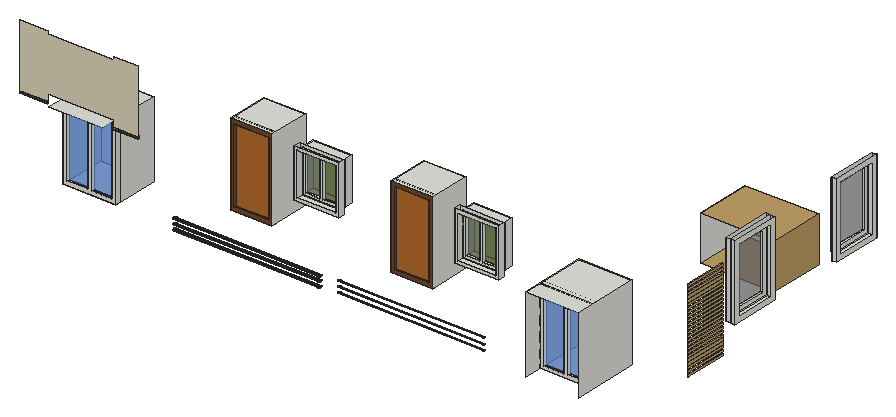
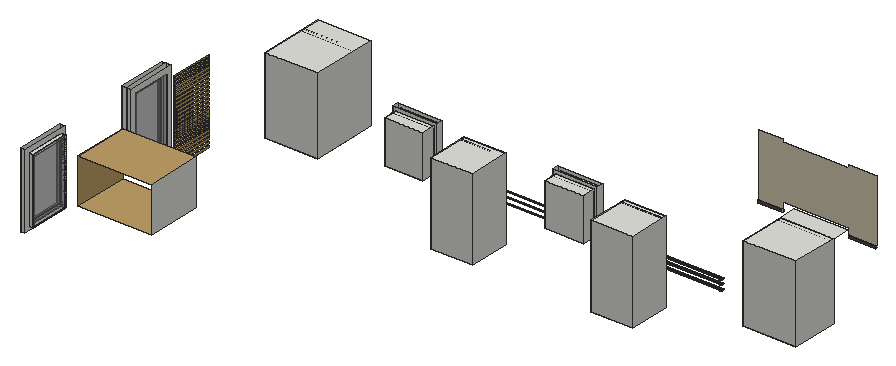
# SketchUp Ruby script. Lengths in inches.
U = 1.inch
M = Sketchup.active_model
def pt(a) = Geom::Point3d.new(a.map { |v| v * U })
def face(e, loops, mat)
  f = e.add_face(loops[0].map { |a| pt(a) })
  loops[1..].each { |l| e.add_face(l.map { |a| pt(a) }).erase! }
  f.material = f.back_material = mat if mat
  f
end
# faces: each face lists its corners as indices into pts; further lists are holes
def faces(e, pts, list, mat = nil) = list.each { |f| face(e, (f[0].is_a?(Array) ? f : [f]).map { |l| l.map { |i| pts[i] } }, mat) }
# xy, xz, yz: faces in a plane at the given z, y or x. An outline is a flat list of corners, or four numbers for a rectangle; further outlines are holes
def ring(l) = l.size == 4 ? [[l[0], l[1]], [l[2], l[1]], [l[2], l[3]], [l[0], l[3]]] : l.each_slice(2).to_a
def flat(e, list, mat, &to3) = list.each { |f| face(e, (f[0].is_a?(Array) ? f : [f]).map { |l| ring(l).map { |u, v| to3.(u, v) } }, mat) }
def xy(e, z, list, mat = nil) = flat(e, list, mat) { |x, y| [x, y, z] }
def xz(e, y, list, mat = nil) = flat(e, list, mat) { |x, z| [x, y, z] }
def yz(e, x, list, mat = nil) = flat(e, list, mat) { |y, z| [x, y, z] }
def lines(e, pts, list) = list.each { |a, b| e.add_line(pt(pts[a]), pt(pts[b])) }
# prism: a flat outline (further loops are holes) pulled along v
def prism(e, loops, v, mat = nil)
  f = face(e, loops, mat); d = Geom::Vector3d.new(v.map { |x| x * U })
  f.pushpull(f.normal.samedirection?(d) ? d.length : -d.length)
end
def box(e, o, s, mat = nil) = prism(e, [[o, [o[0] + s[0], o[1], o[2]], [o[0] + s[0], o[1] + s[1], o[2]], [o[0], o[1] + s[1], o[2]]]], [0, 0, s[2]], mat)
def at(x, y, z, deg = 0) = Geom::Transformation.translation(pt([x, y, z])) * Geom::Transformation.rotation(ORIGIN, Z_AXIS, deg.degrees)
def axes(o, x, y, z) = Geom::Transformation.new([*x, 0, *y, 0, *z, 0, *pt(o).to_a, 1])
def part(name) = M.definitions.add(name)
# library, detail: a bought-in or finely detailed component or shape, given as its bounding box
def library(name, o, s) = part(name).tap { |d| box(d.entities, o, s) }
def detail(e, o, s) = box(e.add_group.entities, o, s)
def put(e, d, t, mat = nil) = e.add_instance(d, t).tap { |i| i.material = mat if mat }
def group(e, t, mat = nil) = e.add_group.tap { |g| g.transformation = t; g.material = mat if mat }.entities
root = M.entities
M.materials.add("Generic").color = [191, 159, 103]
M.materials.add("Generic\#3").color = [218, 209, 183]
M.materials.add("[Color M06]").color = [86, 86, 86]
M.materials.add("[Translucent Glass Blue]").color = [100, 149, 237]
M.materials["[Translucent Glass Blue]"].alpha = 0.5
M.materials.add("[Translucent Glass Dark Green]").color = [62, 91, 5]
M.materials["[Translucent Glass Dark Green]"].alpha = 0.5
M.materials.add("[Translucent Glass Gray]").color = [128, 128, 128]
M.materials["[Translucent Glass Gray]"].alpha = 0.5
M.materials.add("[Wood Bamboo]").color = [177, 105, 43]
M.materials.add("[Wood Veneer 01]").color = [120, 70, 37]
c1 = part("Group\#5")
xy(c1.entities,0,[[0,0,1,57.75]])
xy(c1.entities,2.57,[[0,0,1,57.75]])
xz(c1.entities,0,[[0,0,1,2.57]])
xz(c1.entities,57.75,[[0,0,1,2.57]])
yz(c1.entities,1,[[0,0,57.75,2.57]])
c2 = part("Group\#4")
xy(c2.entities,0,[[0,0,55.6875,6]],"[Wood Veneer 01]")
xy(c2.entities,4.75,[[4.75,0,50.9375,3]],"[Wood Veneer 01]")
xy(c2.entities,105.5,[[4.75,0,50.9375,3]],"[Wood Veneer 01]")
xy(c2.entities,110.25,[[0,0,55.6875,6]],"[Wood Veneer 01]")
xz(c2.entities,0,[[[0,0,55.6875,110.25],[4.75,4.75,50.9375,105.5]]],"[Wood Veneer 01]")
xz(c2.entities,3,[[4.75,4.75,50.9375,105.5]],"[Wood Bamboo]")
xz(c2.entities,6,[[0,0,55.6875,110.25]],"[Wood Bamboo]")
yz(c2.entities,0,[[0,0,6,110.25]],"[Wood Veneer 01]")
yz(c2.entities,4.75,[[0,4.75,3,105.5]],"[Wood Veneer 01]")
yz(c2.entities,50.9375,[[0,4.75,3,105.5]],"[Wood Veneer 01]")
yz(c2.entities,55.6875,[[0,0,6,110.25]],"[Wood Veneer 01]")
c3 = part("Group\#1")
xy(c3.entities,0,[[0,0,71.4375,6]])
xy(c3.entities,5.26,[[5.26,0,33.09,3],[38.35,0,66.18,3]])
xy(c3.entities,97.49,[[5.26,0,33.09,3],[38.35,0,66.18,3]])
xy(c3.entities,102.75,[[0,0,71.4375,6]])
xz(c3.entities,0,[[[0,0,71.4375,102.75],[38.35,5.26,66.18,97.49],[5.26,5.26,33.09,97.49]]])
xz(c3.entities,3,[[5.26,5.26,33.09,97.49],[38.35,5.26,66.18,97.49]],"[Translucent Glass Blue]")
xz(c3.entities,6,[[0,0,71.4375,102.75]],"[Translucent Glass Blue]")
yz(c3.entities,0,[[0,0,6,102.75]])
yz(c3.entities,5.26,[[0,5.26,3,97.49]])
yz(c3.entities,33.09,[[0,5.26,3,97.49]])
yz(c3.entities,38.35,[[0,5.26,3,97.49]])
yz(c3.entities,66.18,[[0,5.26,3,97.49]])
yz(c3.entities,71.4375,[[0,0,6,102.75]])
c4 = part("Group\#7")
xy(c4.entities,0,[[0,0,6,54.3125]])
xy(c4.entities,5.9,[[3,5.9,6,48.41]])
xy(c4.entities,81.98,[[3,5.9,6,48.41]])
xy(c4.entities,87.88,[[0,0,6,54.3125]])
xz(c4.entities,0,[[0,0,6,87.88]])
xz(c4.entities,5.9,[[3,5.9,6,81.98]])
xz(c4.entities,48.41,[[3,5.9,6,81.98]])
xz(c4.entities,54.3125,[[0,0,6,87.88]])
yz(c4.entities,0,[[0,0,54.3125,87.88]],"[Translucent Glass Gray]")
yz(c4.entities,3,[[5.9,5.9,48.41,81.98]],"[Translucent Glass Gray]")
yz(c4.entities,6,[[[0,0,54.3125,87.88],[5.9,5.9,48.41,81.98]]])
c5 = part("Group\#3")
xy(c5.entities,0,[[0,0,51.8125,6]])
xy(c5.entities,4.04,[[4.04,0,23.89,3],[27.93,0,47.77,3]])
xy(c5.entities,53.71,[[4.04,0,23.89,3],[27.93,0,47.77,3]])
xy(c5.entities,57.75,[[0,0,51.8125,6]])
xz(c5.entities,0,[[[0,0,51.8125,57.75],[4.04,4.04,23.89,53.71],[27.93,4.04,47.77,53.71]]])
xz(c5.entities,3,[[4.04,4.04,23.89,53.71],[27.93,4.04,47.77,53.71]],"[Translucent Glass Dark Green]")
xz(c5.entities,6,[[0,0,51.8125,57.75]],"[Translucent Glass Gray]")
yz(c5.entities,0,[[0,0,6,57.75]])
yz(c5.entities,4.04,[[0,4.04,3,53.71]])
yz(c5.entities,23.89,[[0,4.04,3,53.71]])
yz(c5.entities,27.93,[[0,4.04,3,53.71]])
yz(c5.entities,47.77,[[0,4.04,3,53.71]])
yz(c5.entities,51.8125,[[0,0,6,57.75]])
xy(root,461.3125,[[215.38,158.75,271.07,214.75],[431.19,158.75,486.88,214.75]])
xy(root,467.03,[[49.58,83.8125,121.01,146.5625]])
xy(root,469.69,[[691.41,83.8125,762.85,149.3125]])
xy(root,488.89,[[703.98,338.625,802.875,413.6875]],"Generic")
xy(root,489.97,[[802.875,257.24,809.375,324.36],[809.375,257.24,815.3125,324.36],[809.375,428.47,815.3125,495.59]])
xy(root,496.375,[[802.875,263.64,809.375,317.96],[809.375,263.64,815.3125,317.96],[802.875,434.88,809.375,489.19],[809.375,434.88,815.3125,489.19]])
xy(root,508.8,[[307.73,150.125,367.625,158.75],[523.54,150.125,583.4375,158.75]])
xy(root,512.84,[[311.77,150.125,363.58,158.75],[527.58,150.125,579.39,158.75],[311.77,158.75,363.58,177.1875],[527.58,158.75,579.39,177.1875]])
xy(root,549.89,[[703.98,338.625,802.875,413.6875]],"Generic")
xy(root,567.15,[[4.1875,68.5,40.68,69.9375],[129.91,68.5,162.33,69.9375]])
xy(root,569.78,[[49.58,60.5625,121.01,83.8125],[49.58,83.8125,121.01,146.5625]])
xy(root,570.15,[[4.1875,68.5,40.68,69.9375],[129.91,68.5,162.33,69.9375]])
xy(root,570.59,[[311.77,150.125,363.58,158.75],[527.58,150.125,579.39,158.75],[311.77,158.75,363.58,177.1875],[527.58,158.75,579.39,177.1875]])
xy(root,571.5625,[[215.38,158.75,271.07,214.75],[431.19,158.75,486.88,214.75]])
xy(root,572.44,[[691.41,60.5625,762.85,149.3125]])
xz(root,68.5,[[129.35,567.15,129.91,570.15]])
xz(root,68.5,[[4.1875,570.15,40.68,570.15,40.68,578.68,129.91,578.68,129.91,570.15,162.33,570.15,162.33,655.14,130.34,655.14,130.34,651.7,41.1,651.7,41.1,655.14,4.1875,655.14]],"Generic\#3")
xz(root,69.9375,[[4.1875,567.15,40.68,570.15],[129.91,567.15,162.33,570.15]],"[Color M06]")
xz(root,146.5625,[[49.58,467.03,121.01,569.78]])
xz(root,149.3125,[[691.41,469.69,762.85,572.44]])
xz(root,150.125,[[[307.73,508.8,367.625,574.63],[311.77,512.84,363.58,570.59]],[[523.54,508.8,583.4375,574.63],[527.58,512.84,579.39,570.59]]])
xz(root,158.75,[[[307.73,508.8,367.625,574.63],[311.77,512.84,363.58,570.59]],[[523.54,508.8,583.4375,574.63],[527.58,512.84,579.39,570.59]]])
xz(root,177.1875,[[311.77,512.84,363.58,570.59],[527.58,512.84,579.39,570.59]])
xz(root,214.75,[[215.38,461.3125,271.07,571.5625],[431.19,461.3125,486.88,571.5625]])
xz(root,257.24,[[802.875,489.97,809.375,590.66],[809.375,489.97,815.3125,590.66]])
xz(root,263.64,[[802.875,496.375,809.375,584.25],[809.375,496.375,815.3125,584.25]])
xz(root,317.96,[[802.875,496.375,809.375,584.25],[809.375,496.375,815.3125,584.25]])
xz(root,324.36,[[802.875,489.97,809.375,590.66],[809.375,489.97,815.3125,590.66]])
xz(root,428.47,[[809.375,489.97,815.3125,590.66]])
xz(root,434.88,[[802.875,496.375,809.375,584.25],[809.375,496.375,815.3125,584.25]])
xz(root,489.19,[[802.875,496.375,809.375,584.25],[809.375,496.375,815.3125,584.25]])
xz(root,495.59,[[809.375,489.97,815.3125,590.66]])
yz(root,49.58,[[83.8125,467.03,146.5625,569.78]])
yz(root,121.01,[[83.8125,467.03,146.5625,569.78]])
yz(root,129.91,[[68.5,567.15,69.9375,570.15]])
yz(root,215.38,[[158.75,461.3125,214.75,571.5625]])
yz(root,271.07,[[158.75,461.3125,214.75,571.5625]])
yz(root,307.73,[[150.125,508.8,158.75,574.63]])
yz(root,311.77,[[150.125,512.84,158.75,570.59],[158.75,512.84,177.1875,570.59]])
yz(root,363.58,[[150.125,512.84,158.75,570.59],[158.75,512.84,177.1875,570.59]])
yz(root,367.625,[[150.125,508.8,158.75,574.63]])
yz(root,431.19,[[158.75,461.3125,214.75,571.5625]])
yz(root,486.88,[[158.75,461.3125,214.75,571.5625]])
yz(root,523.54,[[150.125,508.8,158.75,574.63]])
yz(root,527.58,[[150.125,512.84,158.75,570.59],[158.75,512.84,177.1875,570.59]])
yz(root,579.39,[[150.125,512.84,158.75,570.59],[158.75,512.84,177.1875,570.59]])
yz(root,583.4375,[[150.125,508.8,158.75,574.63]])
yz(root,691.41,[[60.5625,469.69,149.3125,572.44]])
yz(root,703.98,[[338.625,488.89,413.6875,549.89]])
yz(root,762.85,[[60.5625,469.69,149.3125,572.44]])
yz(root,802.875,[[[257.24,489.97,324.36,590.66],[263.64,496.375,317.96,584.25]]])
yz(root,802.875,[[338.625,488.89,413.6875,549.89]],"Generic")
yz(root,809.375,[[[257.24,489.97,324.36,590.66],[263.64,496.375,317.96,584.25]],[[428.47,489.97,495.59,590.66],[434.88,496.375,489.19,584.25]]])
yz(root,815.3125,[[[257.24,489.97,324.36,590.66],[263.64,496.375,317.96,584.25]],[[428.47,489.97,495.59,590.66],[434.88,496.375,489.19,584.25]]])
p = [[193.83,89.44,458.87],[193.83,89.73,458.75],[391.53,89.73,458.75],[391.53,89.44,458.87],[193.83,90.04,458.71],[391.53,90.04,458.71],
  [193.83,90.35,458.75],[391.53,90.35,458.75],[193.83,90.63,458.87],[391.53,90.63,458.87],[193.83,89.2,459.06],[391.53,89.2,459.06],
  [193.83,90.88,459.06],[391.53,90.88,459.06],[193.83,89.01,459.3],[391.53,89.01,459.3],[193.83,91.07,459.3],[391.53,91.07,459.3],
  [193.83,88.89,459.59],[391.53,88.89,459.59],[193.83,91.18,459.59],[391.53,91.18,459.59],[193.83,88.85,459.9],[391.53,88.85,459.9],
  [193.83,91.23,459.9],[391.53,91.23,459.9],[193.83,88.89,460.2],[391.53,88.89,460.2],[193.83,91.18,460.2],[391.53,91.18,460.2],
  [193.83,89.01,460.49],[391.53,89.01,460.49],[193.83,91.07,460.49],[391.53,91.07,460.49],[193.83,89.2,460.74],[391.53,89.2,460.74],
  [193.83,90.88,460.74],[391.53,90.88,460.74],[193.83,89.44,460.92],[391.53,89.44,460.92],[193.83,90.63,460.92],[391.53,90.63,460.92],
  [193.83,89.73,461.04],[391.53,89.73,461.04],[193.83,90.35,461.04],[391.53,90.35,461.04],[193.83,90.04,461.08],[391.53,90.04,461.08],
  [415.53,89.0625,461.17],[415.53,89.21,461.15],[613.23,89.21,461.15],[613.23,89.0625,461.17],[415.53,89.36,461.17],[613.23,89.36,461.17],
  [415.53,88.8125,461.3125],[415.53,88.93,461.22],[613.23,88.93,461.22],[613.23,88.8125,461.3125],[415.53,89.49,461.22],[613.23,89.49,461.22],
  [415.53,89.61,461.3125],[613.23,89.61,461.3125],[415.53,88.72,461.43],[613.23,88.72,461.43],[415.53,89.7,461.43],[613.23,89.7,461.43],
  [415.53,88.67,461.57],[613.23,88.67,461.57],[415.53,89.75,461.57],[613.23,89.75,461.57],[415.53,88.65,461.71],[613.23,88.65,461.71],
  [415.53,89.77,461.71],[613.23,89.77,461.71],[415.53,88.67,461.86],[613.23,88.67,461.86],[415.53,89.75,461.86],[613.23,89.75,461.86],
  [415.53,88.72,461.99],[613.23,88.72,461.99],[415.53,89.7,461.99],[613.23,89.7,461.99],[415.53,88.8125,462.11],[613.23,88.8125,462.11],
  [415.53,89.61,462.11],[613.23,89.61,462.11],[415.53,88.93,462.2],[613.23,88.93,462.2],[415.53,89.49,462.2],[613.23,89.49,462.2],
  [415.53,89.0625,462.26],[613.23,89.0625,462.26],[415.53,89.36,462.26],[613.23,89.36,462.26],[415.53,89.21,462.27],[613.23,89.21,462.27],
  [193.83,89.44,465.87],[193.83,89.73,465.75],[391.53,89.73,465.75],[391.53,89.44,465.87],[193.83,90.04,465.71],[391.53,90.04,465.71],
  [193.83,90.35,465.75],[391.53,90.35,465.75],[193.83,90.63,465.87],[391.53,90.63,465.87],[193.83,89.2,466.06],[391.53,89.2,466.06],
  [193.83,90.88,466.06],[391.53,90.88,466.06],[193.83,89.01,466.3],[391.53,89.01,466.3],[193.83,91.07,466.3],[391.53,91.07,466.3],
  [193.83,88.89,466.59],[391.53,88.89,466.59],[193.83,91.18,466.59],[391.53,91.18,466.59],[193.83,88.85,466.9],[391.53,88.85,466.9],
  [193.83,91.23,466.9],[391.53,91.23,466.9],[193.83,88.89,467.2],[391.53,88.89,467.2],[193.83,91.18,467.2],[391.53,91.18,467.2],
  [193.83,89.01,467.49],[391.53,89.01,467.49],[193.83,91.07,467.49],[391.53,91.07,467.49],[193.83,89.2,467.74],[391.53,89.2,467.74],
  [193.83,90.88,467.74],[391.53,90.88,467.74],[193.83,89.44,467.92],[391.53,89.44,467.92],[193.83,90.63,467.92],[391.53,90.63,467.92],
  [193.83,89.73,468.04],[391.53,89.73,468.04],[193.83,90.35,468.04],[391.53,90.35,468.04],[193.83,90.04,468.08],[391.53,90.04,468.08],
  [415.53,89.0625,468.67],[415.53,89.21,468.65],[613.23,89.21,468.65],[613.23,89.0625,468.67],[415.53,89.36,468.67],[613.23,89.36,468.67],
  [415.53,88.8125,468.8125],[415.53,88.93,468.72],[613.23,88.93,468.72],[613.23,88.8125,468.8125],[415.53,89.49,468.72],[613.23,89.49,468.72],
  [415.53,89.61,468.8125],[613.23,89.61,468.8125],[415.53,88.72,468.93],[613.23,88.72,468.93],[415.53,89.7,468.93],[613.23,89.7,468.93],
  [415.53,88.67,469.07],[613.23,88.67,469.07],[415.53,89.75,469.07],[613.23,89.75,469.07],[415.53,88.65,469.21],[613.23,88.65,469.21],
  [415.53,89.77,469.21],[613.23,89.77,469.21],[415.53,88.67,469.36],[613.23,88.67,469.36],[415.53,89.75,469.36],[613.23,89.75,469.36],
  [415.53,88.72,469.49],[613.23,88.72,469.49],[415.53,89.7,469.49],[613.23,89.7,469.49],[415.53,88.8125,469.61],[613.23,88.8125,469.61],
  [415.53,89.61,469.61],[613.23,89.61,469.61],[415.53,88.93,469.7],[613.23,88.93,469.7],[415.53,89.49,469.7],[613.23,89.49,469.7],
  [415.53,89.0625,469.76],[613.23,89.0625,469.76],[415.53,89.36,469.76],[613.23,89.36,469.76],[415.53,89.21,469.77],[613.23,89.21,469.77],
  [193.83,89.44,472.43],[193.83,89.73,472.3125],[391.53,89.73,472.3125],[391.53,89.44,472.43],[193.83,90.04,472.27],[391.53,90.04,472.27],
  [193.83,90.35,472.3125],[391.53,90.35,472.3125],[193.83,90.63,472.43],[391.53,90.63,472.43],[193.83,89.2,472.62],[391.53,89.2,472.62],
  [193.83,90.88,472.62],[391.53,90.88,472.62],[193.83,89.01,472.86],[391.53,89.01,472.86],[193.83,91.07,472.86],[391.53,91.07,472.86],
  [193.83,88.89,473.15],[391.53,88.89,473.15],[193.83,91.18,473.15],[391.53,91.18,473.15],[193.83,88.85,473.46],[391.53,88.85,473.46],
  [193.83,91.23,473.46],[391.53,91.23,473.46],[193.83,88.89,473.77],[391.53,88.89,473.77],[193.83,91.18,473.77],[391.53,91.18,473.77],
  [193.83,89.01,474.05],[391.53,89.01,474.05],[193.83,91.07,474.05],[391.53,91.07,474.05],[193.83,89.2,474.3],[391.53,89.2,474.3],
  [193.83,90.88,474.3],[391.53,90.88,474.3],[193.83,89.44,474.49],[391.53,89.44,474.49],[193.83,90.63,474.49],[391.53,90.63,474.49],
  [193.83,89.73,474.61],[391.53,89.73,474.61],[193.83,90.35,474.61],[391.53,90.35,474.61],[193.83,90.04,474.65],[391.53,90.04,474.65],
  [415.53,88.93,476.16],[415.53,89.0625,476.11],[613.23,89.0625,476.11],[613.23,88.93,476.16],[415.53,89.21,476.09],[613.23,89.21,476.09],
  [415.53,89.36,476.11],[613.23,89.36,476.11],[415.53,89.49,476.16],[613.23,89.49,476.16],[415.53,88.8125,476.25],[613.23,88.8125,476.25],
  [415.53,89.61,476.25],[613.23,89.61,476.25],[415.53,88.72,476.37],[613.23,88.72,476.37],[415.53,89.7,476.37],[613.23,89.7,476.37],
  [415.53,88.67,476.5],[613.23,88.67,476.5],[415.53,89.75,476.5],[613.23,89.75,476.5],[415.53,88.65,476.65],[613.23,88.65,476.65],
  [415.53,89.77,476.65],[613.23,89.77,476.65],[415.53,88.67,476.79],[613.23,88.67,476.79],[415.53,89.75,476.79],[613.23,89.75,476.79],
  [415.53,88.72,476.93],[613.23,88.72,476.93],[415.53,89.7,476.93],[613.23,89.7,476.93],[415.53,88.8125,477.05],[613.23,88.8125,477.05],
  [415.53,89.61,477.05],[613.23,89.61,477.05],[415.53,88.93,477.14],[613.23,88.93,477.14],[415.53,89.49,477.14],[613.23,89.49,477.14],
  [415.53,89.0625,477.19],[613.23,89.0625,477.19],[415.53,89.36,477.19],[613.23,89.36,477.19],[415.53,89.21,477.21],[613.23,89.21,477.21],
  [415.53,89.21,476.68],[613.23,89.21,476.68],[415.53,89.21,461.81],[613.23,89.21,461.81],[415.53,89.21,469.24],[613.23,89.21,469.24],
  [193.83,90.04,473.27],[391.53,90.04,473.27],[193.83,90.04,459.77],[391.53,90.04,459.77],[193.83,90.04,466.52],[391.53,90.04,466.52]]
faces(root,p,[[0,1,2,3],[1,4,5,2],[4,6,7,5],[6,8,9,7],[10,0,3,11],[8,12,13,9],[14,10,11,15],[12,16,17,13],
  [18,14,15,19],[16,20,21,17],[22,18,19,23],[20,24,25,21],[26,22,23,27],[24,28,29,25],[30,26,27,31],[28,32,33,29],
  [34,30,31,35],[32,36,37,33],[38,34,35,39],[36,40,41,37],[42,38,39,43],[40,44,45,41],[46,42,43,47],[44,46,47,45],
  [48,49,50,51],[49,52,53,50],[54,55,56,57],[55,48,51,56],[52,58,59,53],[58,60,61,59],[62,54,57,63],[60,64,65,61],
  [66,62,63,67],[64,68,69,65],[70,66,67,71],[68,72,73,69],[74,70,71,75],[72,76,77,73],[78,74,75,79],[76,80,81,77],
  [82,78,79,83],[80,84,85,81],[86,82,83,87],[84,88,89,85],[90,86,87,91],[88,92,93,89],[94,90,91,95],[92,94,95,93],
  [96,97,98,99],[97,100,101,98],[100,102,103,101],[102,104,105,103],[106,96,99,107],[104,108,109,105],[110,106,107,111],[108,112,113,109],
  [114,110,111,115],[112,116,117,113],[118,114,115,119],[116,120,121,117],[122,118,119,123],[120,124,125,121],[126,122,123,127],[124,128,129,125],
  [130,126,127,131],[128,132,133,129],[134,130,131,135],[132,136,137,133],[138,134,135,139],[136,140,141,137],[142,138,139,143],[140,142,143,141],
  [144,145,146,147],[145,148,149,146],[150,151,152,153],[151,144,147,152],[148,154,155,149],[154,156,157,155],[158,150,153,159],[156,160,161,157],
  [162,158,159,163],[160,164,165,161],[166,162,163,167],[164,168,169,165],[170,166,167,171],[168,172,173,169],[174,170,171,175],[172,176,177,173],
  [178,174,175,179],[176,180,181,177],[182,178,179,183],[180,184,185,181],[186,182,183,187],[184,188,189,185],[190,186,187,191],[188,190,191,189],
  [192,193,194,195],[193,196,197,194],[196,198,199,197],[198,200,201,199],[202,192,195,203],[200,204,205,201],[206,202,203,207],[204,208,209,205],
  [210,206,207,211],[208,212,213,209],[214,210,211,215],[212,216,217,213],[218,214,215,219],[216,220,221,217],[222,218,219,223],[220,224,225,221],
  [226,222,223,227],[224,228,229,225],[230,226,227,231],[228,232,233,229],[234,230,231,235],[232,236,237,233],[238,234,235,239],[236,238,239,237],
  [240,241,242,243],[241,244,245,242],[244,246,247,245],[246,248,249,247],[250,240,243,251],[248,252,253,249],[254,250,251,255],[252,256,257,253],
  [258,254,255,259],[256,260,261,257],[262,258,259,263],[260,264,265,261],[266,262,263,267],[264,268,269,265],[270,266,267,271],[268,272,273,269],
  [274,270,271,275],[272,276,277,273],[278,274,275,279],[276,280,281,277],[282,278,279,283],[280,284,285,281],[286,282,283,287],[284,286,287,285]])
lines(root,p,[[288,289],[290,291],[292,293],[294,295],[296,297],[298,299]])
put(root,c1,at(809.375,185.01,456.33),"Generic")
put(root,c1,at(809.375,185.01,461.08),"Generic")
put(root,c2,at(431.19,158.75,461.3125))
put(root,c2,at(215.38,158.75,461.3125))
put(root,c1,at(809.375,185.01,465.83),"Generic")
put(root,c3,at(49.58,83.8125,467.03))
put(root,c3,at(691.41,83.8125,469.69))
put(root,c1,at(809.375,185.01,470.58),"Generic")
put(root,c1,at(809.375,185.01,475.33),"Generic")
put(root,c1,at(809.375,185.01,480.08),"Generic")
put(root,c1,at(809.375,185.01,484.83),"Generic")
put(root,c1,at(809.375,185.01,489.58),"Generic")
put(root,c1,at(809.375,185.01,494.33),"Generic")
put(root,c4,at(803.375,434.88,496.375))
put(root,c4,at(803.375,263.64,496.375))
put(root,c1,at(809.375,185.01,499.08),"Generic")
put(root,c1,at(809.375,185.01,503.83),"Generic")
put(root,c1,at(809.375,185.01,508.58),"Generic")
put(root,c5,at(311.77,158.75,512.84))
put(root,c5,at(527.58,158.75,512.84))
put(root,c1,at(809.375,185.01,513.33),"Generic")
put(root,c1,at(809.375,185.01,518.08),"Generic")
put(root,c1,at(809.375,185.01,522.83),"Generic")
put(root,c1,at(809.375,185.01,527.58),"Generic")
put(root,c1,at(809.375,185.01,532.33),"Generic")
put(root,c1,at(809.375,185.01,537.08),"Generic")
put(root,c1,at(809.375,185.01,541.83),"Generic")
put(root,c1,at(809.375,185.01,546.58),"Generic")
put(root,c1,at(809.375,185.01,551.33),"Generic")
put(root,c1,at(809.375,185.01,556.08),"Generic")
put(root,c1,at(809.375,185.01,560.83),"Generic")
put(root,c1,at(809.375,185.01,565.58),"Generic")
